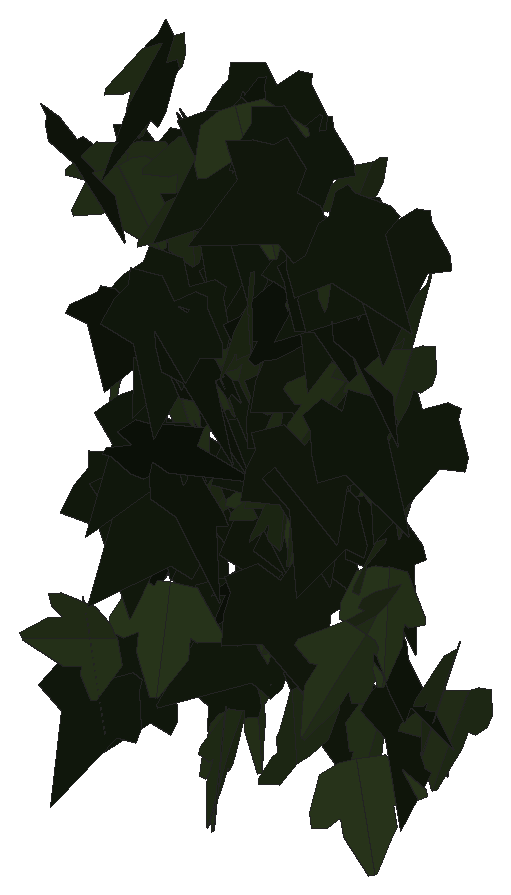
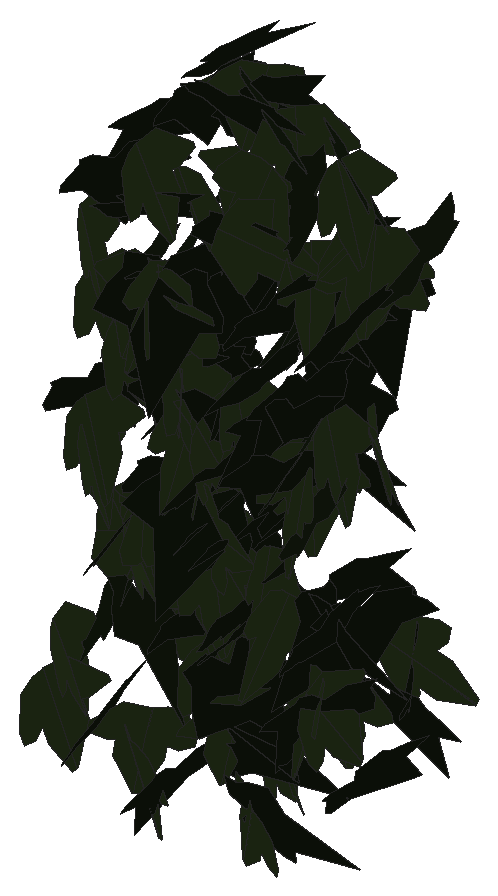
# SketchUp Ruby script. Lengths in inches.
U = 1.inch
M = Sketchup.active_model
def pt(a) = Geom::Point3d.new(a.map { |v| v * U })
def face(e, loops, mat)
  f = e.add_face(loops[0].map { |a| pt(a) })
  loops[1..].each { |l| e.add_face(l.map { |a| pt(a) }).erase! }
  f.material = f.back_material = mat if mat
  f
end
# faces: each face lists its corners as indices into pts; further lists are holes
def faces(e, pts, list, mat = nil) = list.each { |f| face(e, (f[0].is_a?(Array) ? f : [f]).map { |l| l.map { |i| pts[i] } }, mat) }
# xy, xz, yz: faces in a plane at the given z, y or x. An outline is a flat list of corners, or four numbers for a rectangle; further outlines are holes
def ring(l) = l.size == 4 ? [[l[0], l[1]], [l[2], l[1]], [l[2], l[3]], [l[0], l[3]]] : l.each_slice(2).to_a
def flat(e, list, mat, &to3) = list.each { |f| face(e, (f[0].is_a?(Array) ? f : [f]).map { |l| ring(l).map { |u, v| to3.(u, v) } }, mat) }
def xy(e, z, list, mat = nil) = flat(e, list, mat) { |x, y| [x, y, z] }
def xz(e, y, list, mat = nil) = flat(e, list, mat) { |x, z| [x, y, z] }
def yz(e, x, list, mat = nil) = flat(e, list, mat) { |y, z| [x, y, z] }
def lines(e, pts, list) = list.each { |a, b| e.add_line(pt(pts[a]), pt(pts[b])) }
# prism: a flat outline (further loops are holes) pulled along v
def prism(e, loops, v, mat = nil)
  f = face(e, loops, mat); d = Geom::Vector3d.new(v.map { |x| x * U })
  f.pushpull(f.normal.samedirection?(d) ? d.length : -d.length)
end
def box(e, o, s, mat = nil) = prism(e, [[o, [o[0] + s[0], o[1], o[2]], [o[0] + s[0], o[1] + s[1], o[2]], [o[0], o[1] + s[1], o[2]]]], [0, 0, s[2]], mat)
def at(x, y, z, deg = 0) = Geom::Transformation.translation(pt([x, y, z])) * Geom::Transformation.rotation(ORIGIN, Z_AXIS, deg.degrees)
def axes(o, x, y, z) = Geom::Transformation.new([*x, 0, *y, 0, *z, 0, *pt(o).to_a, 1])
def part(name) = M.definitions.add(name)
# library, detail: a bought-in or finely detailed component or shape, given as its bounding box
def library(name, o, s) = part(name).tap { |d| box(d.entities, o, s) }
def detail(e, o, s) = box(e.add_group.entities, o, s)
def put(e, d, t, mat = nil) = e.add_instance(d, t).tap { |i| i.material = mat if mat }
def group(e, t, mat = nil) = e.add_group.tap { |g| g.transformation = t; g.material = mat if mat }.entities
root = M.entities
M.materials.add("efeu1").color = [18, 25, 13]
M.materials.add("efeu2").color = [43, 57, 29]
c1 = part("ivyleaf_10")
p = [[0,0.5,-0.03],[-0.0625,2.02,-0.43],[-0.19,2.01,-0.46],[-0.54,1.05,-0.29],[-0.52,0.625,-0.18],[-0.83,0.76,-0.28],
  [-1.16,0.64,-0.33],[-1.15,0.33,-0.24],[-0.77,-0.39,0.02],[-0.3,-0.51,0.16],[0.04,-0.48,0.23],[-0.02,2.01,-0.4375],
  [-0.06,2.01,-0.43],[0.04,-0.49,0.23],[0.67,-0.49,0.14],[1.38,0.36,-0.2],[1.375,0.51,-0.24],[0.81,0.65,-0.19],
  [0.62,0.59,-0.15],[0.6,1.09,-0.28],[0.5,1.23,-0.31]]
faces(c1.entities,p,[[0,1,2,3,4,5,6,7,8,9,10],[11,12,0,13,14,15,16,17,18,19,20]],"efeu2")
c2 = part("ivyleaf_9")
p = [[1.54,2.16,1.25],[1.36,2.04,1.19],[-0.21,0.99,0.68],[-0.71,1.11,0.82],[-0.85,0.86,0.67],[-0.8,0.17,0.21],
  [-0.9,-0.01,0.1],[-0.67,-0.16,-0.02],[-0.08,-0.08,-0.05],[-0.03,-0.6,-0.4],[0.65,-0.88,-0.66],[0.83,-0.6,-0.49],
  [1.29,-0.42,-0.43],[1.8125,-0.07,-0.26],[1.21,0.44,0.15]]
faces(c2.entities,p,[[0,1,2,3,4,5,6,7,8,9,10,11,12,13,14]],"efeu1")
put(root,c1,axes([10.84,223.45,235.51],[0.02548,-0.41018,0.28478],[0.04221,-0.28236,-0.41048],[0.49756,0.04496,0.02023]))
put(root,c2,axes([10.51,222.08,240.66],[0.18822,-0.39499,0.24198],[0.16985,-0.18415,-0.43271],[0.43096,0.24509,0.06485]))
put(root,c1,axes([10.89,223.15,238.77],[0.04724,-0.49773,-0.006],[-0.00088,0.00594,-0.49996],[0.49776,0.04725,-0.00031]))
put(root,c1,axes([11.29,221.38,235.1875],[0.17508,0.01809,-0.46799],[-0.45924,0.10468,-0.16776],[0.09191,0.48858,0.05327]))
put(root,c2,axes([11.35,222.68,236.02],[-0.27745,0.22546,0.34956],[-0.26223,0.23136,-0.35736],[-0.32289,-0.38163,-0.01014]))
put(root,c1,axes([10.84,222.45,238.39],[0.34561,-0.29172,0.2132],[0.16573,-0.13418,-0.45225],[0.32107,0.38327,0.00395]))
put(root,c2,axes([10.78,223.09,240.23],[0.09676,-0.48882,-0.0412],[-0.00215,0.04157,-0.49826],[0.49054,0.0966,0.00594]))
put(root,c2,axes([10.89,222.64,236.41],[-0.18069,-0.44824,-0.12818],[0.05611,0.11556,-0.48322],[0.46282,-0.18901,0.00854]))
put(root,c2,axes([10.79,223.46,235.625],[0.0421,-0.43866,-0.23623],[0.04754,0.23953,-0.43631],[0.49595,0.01428,0.06188]))
put(root,c1,axes([11.03,223.36,235.61],[-0.38254,0.31627,0.06032],[-0.04509,0.04013,-0.49634],[-0.3188,-0.38518,-0.00218]))
put(root,c2,axes([11,222.59,234.2],[-0.18711,-0.40957,0.21735],[-0.052,-0.21436,-0.44871],[0.46074,-0.19053,0.03762]))
put(root,c2,axes([10.9,223.36,236.46],[0.01066,-0.49178,0.08967],[-0.01623,-0.08999,-0.49157],[0.49962,0.00757,-0.01788]))
put(root,c1,axes([11.12,222.19,240.65],[-0.39827,-0.30148,-0.02208],[0.01989,0.0103,-0.4995],[0.30163,-0.39875,0.00379]))
put(root,c1,axes([11.14,222.65,241.67],[-0.03559,-0.49633,0.04884],[0.00728,-0.04948,-0.49749],[0.49868,-0.0347,0.01075]))
put(root,c1,axes([11.11,222.17,240.39],[-0.35194,-0.31525,-0.16357],[0.14773,0.07947,-0.47102],[0.32297,-0.37987,0.03721]))
put(root,c2,axes([11.36,222.57,236.07],[-0.06999,0.10256,-0.48434],[-0.28778,0.3896,0.12408],[0.40285,0.29613,0.00449]))
put(root,c2,axes([11.01,223.32,237.77],[0.07513,-0.36679,0.33139],[0.13299,-0.30784,-0.37087],[0.4761,0.14387,0.0513]))
put(root,c2,axes([11.7,223.52,233.92],[-0.31021,0.15343,0.36087],[-0.32922,0.14808,-0.34596],[-0.21303,-0.45225,0.00915]))
put(root,c2,axes([11.37,221.51,234.61],[-0.45437,-0.12225,-0.16912],[0.1684,0.02449,-0.47015],[0.12324,-0.48421,0.01892]))
put(root,c1,axes([11.47,223.05,237.92],[-0.41018,0.24847,0.14148],[-0.12293,0.07011,-0.47955],[-0.25814,-0.42819,0.00357]))
put(root,c2,axes([11.48,222.32,241.83],[-0.42375,0.15045,-0.21864],[0.20508,-0.07586,-0.44965],[-0.16847,-0.47076,0.00259]))
put(root,c1,axes([11.53,222.84,238.07],[-0.421,-0.25867,0.07647],[-0.06549,-0.03947,-0.49412],[0.26166,-0.42607,-0.00065]))
put(root,c1,axes([11.34,222.52,235.1],[0.47007,0.17038,0.00269],[0.00214,0.00197,-0.49999],[-0.17039,0.47007,0.00112]))
put(root,c2,axes([11.5,222.37,236.4],[-0.26805,-0.37411,0.19543],[-0.06401,-0.1928,-0.45687],[0.4172,-0.26994,0.05546]))
put(root,c2,axes([11.34,223.1,239.26],[0.10277,-0.38413,-0.30312],[-0.06428,0.29645,-0.39747],[0.48508,0.12067,0.01155]))
put(root,c2,axes([11.2,221.4,235.17],[0.10419,-0.08708,-0.48121],[0.46944,-0.12002,0.12336],[-0.13699,-0.47751,0.05674]))
put(root,c1,axes([11.54,223.25,236.35],[-0.07687,-0.38054,-0.31508],[0.11176,0.29721,-0.38623],[0.48125,-0.12981,0.03936]))
put(root,c2,axes([11.45,223.21,238.9375],[0.09899,-0.3626,-0.32973],[0.0401,0.34125,-0.36323],[0.48846,0.04547,0.09665]))
put(root,c2,axes([11.53,223.23,238.24],[-0.1301,-0.41783,-0.24186],[0.10378,0.22043,-0.43662],[0.47149,-0.16381,0.02937]))
put(root,c2,axes([11.82,221.88,237.74],[-0.48579,-0.0778,-0.08917],[0.09055,-0.00181,-0.49173],[0.07619,-0.49391,0.01585]))
put(root,c2,axes([11.52,223.19,238.13],[0.03974,-0.3783,0.32452],[0.03619,-0.3225,-0.38038],[0.4971,0.05372,0.00175]))
put(root,c1,axes([11.68,222.3125,238.125],[-0.48655,0.04075,-0.10777],[0.10295,-0.05621,-0.48605],[-0.05173,-0.49516,0.04631]))
put(root,c2,axes([11.96,223.44,234.66],[-0.44214,-0.18738,0.13927],[-0.1315,-0.04659,-0.48014],[0.19292,-0.46121,-0.00808]))
put(root,c1,axes([11.77,223.1875,236.82],[0.04076,-0.43502,-0.24311],[0.03143,0.24568,-0.43434],[0.49734,0.02012,0.04737]))
put(root,c1,axes([11.81,222.37,240.28],[-0.10591,-0.47674,-0.10723],[0.01577,0.10633,-0.48831],[0.4884,-0.10681,-0.00748]))
put(root,c1,axes([11.67,223.57,233.89],[0.36571,-0.17378,0.29335],[0.27919,-0.09433,-0.40393],[0.19573,0.45924,0.02804]))
put(root,c2,axes([12.04,221.09,239.6],[0.22806,0.29386,-0.33412],[-0.20359,-0.26493,-0.37197],[-0.39565,0.30572,-0.00119]))
put(root,c2,axes([12.14,223.38,235.53],[-0.14157,0.39536,-0.27138],[-0.00204,-0.28346,-0.41188],[-0.47954,-0.11551,0.08187]))
put(root,c2,axes([11.9,223.06,240.01],[-0.06871,-0.48727,0.0886],[-0.00063,-0.08936,-0.49195],[0.49526,-0.06772,0.01167]))
put(root,c2,axes([12.25,223.34,235.95],[-0.11499,-0.48033,0.07788],[0.01734,0.07593,0.4939],[-0.48629,0.11629,-0.00081]))
put(root,c2,axes([11.84,222.38,241.13],[0.44335,-0.22332,-0.05972],[-0.05211,0.0293,-0.49641],[0.22522,0.4464,0.00271]))
put(root,c1,axes([12.42,222.86,240.65],[0.14389,0.08329,-0.47155],[-0.47746,-0.01255,-0.14791],[-0.03647,0.49285,0.07593]))
put(root,c1,axes([12.01,223.44,235.1],[0.16365,0.46864,0.05992],[0.00654,0.06116,-0.4962],[-0.47241,0.16319,0.01389]))
put(root,c2,axes([12.17,221.84,239.54],[-0.40783,-0.26544,-0.11495],[0.10084,0.05578,-0.48654],[0.27112,-0.42003,0.00804]))
put(root,c1,axes([12.5625,223.24,237.01],[0.08937,-0.00659,0.4919],[-0.48188,0.09947,0.08888],[-0.09903,-0.48996,0.01143]))
put(root,c2,axes([12.05,223.01,239.15],[0.15848,-0.43802,-0.18173],[-0.02721,0.18289,-0.46455],[0.47344,0.15714,0.03414]))
put(root,c1,axes([12.34,222.97,238.65],[0.03883,-0.49819,-0.01743],[0.00051,0.01752,-0.49969],[0.49849,0.03878,0.00187]))
put(root,c2,axes([12.2,223.34,235.86],[-0.0899,-0.44301,0.21367],[0.00605,-0.21819,-0.44984],[0.49182,-0.07829,0.04459]))
put(root,c1,axes([12.39,223.4,235.54],[-0.20066,-0.41968,0.18331],[-0.00122,-0.19964,-0.45841],[0.45797,-0.18442,0.07909]))
put(root,c2,axes([12.21,223.23,237.07],[0.02918,-0.49184,-0.08508],[0.01466,0.08603,-0.49232],[0.49893,0.02624,0.01944]))
put(root,c1,axes([12.47,223.26,236.625],[-0.15938,-0.47378,0.01133],[-0.0037,-0.01071,-0.49987],[0.4739,-0.15942,-0.0001]))
put(root,c1,axes([12.35,222.62,241.22],[-0.46665,0.10009,-0.14905],[0.13531,-0.07676,-0.47518],[-0.11801,-0.48383,0.04456]))
put(root,c1,axes([12.24,222.31,233.93],[0.29802,-0.249,0.31493],[0.25425,-0.18649,-0.38804],[0.31071,0.39143,0.01545]))
put(root,c2,axes([12.19,220.99,238.03],[0.42036,0.15167,0.22427],[0.20486,0.0926,-0.44661],[-0.17701,0.46735,0.01571]))
put(root,c1,axes([12.52,223.24,236.64],[-0.32542,-0.37456,0.06166],[0.02624,-0.10322,-0.48853],[0.3787,-0.31472,0.08683]))
put(root,c1,axes([12.54,221.75,241.45],[-0.28648,-0.40978,-0.00337],[0.00194,0.00276,-0.49999],[0.40979,-0.28648,0]))
put(root,c1,axes([12.41,222.31,234.01],[0.12891,-0.40923,0.25674],[0.1434,-0.22133,-0.42479],[0.46132,0.18315,0.06031]))
put(root,c2,axes([12.47,222.76,240.62],[-0.34704,-0.2344,-0.27316],[0.22642,0.1528,-0.41879],[0.27981,-0.41438,0.00009]))
put(root,c2,axes([12.3,221.65,237.35],[0.19597,-0.44556,0.11432],[0.05896,-0.0989,-0.48656],[0.4562,0.20418,0.01378]))
put(root,c2,axes([12.51,221.19,239.75],[-0.087,-0.49152,0.0289],[0.0062,-0.03043,-0.49903],[0.49233,-0.08648,0.01139]))
put(root,c2,axes([12.66,223.2,237.4],[0.30201,0.39839,-0.00861],[-0.05714,0.0326,-0.49565],[-0.39437,0.30037,0.06522]))
put(root,c1,axes([12.73,223.1,236.92],[-0.06092,-0.49148,0.06879],[-0.01639,-0.06728,-0.49518],[0.496,-0.06259,-0.00792]))
put(root,c1,axes([12.72,223.06,238.03],[0.07347,-0.44124,0.22341],[0.05732,-0.21675,-0.44692],[0.49124,0.09129,0.01874]))
put(root,c2,axes([12.53,223.19,237.82],[0.12921,-0.46086,-0.14462],[-0.00778,0.1477,-0.47762],[0.48295,0.12568,0.031]))
put(root,c2,axes([12.49,221.39,239.08],[0.35007,-0.35578,-0.02955],[-0.01918,0.02259,-0.49912],[0.35649,0.35059,0.00217]))
put(root,c2,axes([12.51,221.35,239.27],[0.27087,-0.41733,0.04961],[0.03053,-0.03933,-0.49751],[0.41916,0.27255,0.00418]))
put(root,c2,axes([12.67,222.18,241.89],[-0.30074,-0.12828,-0.37828],[0.39862,-0.12679,-0.27392],[-0.02564,-0.46634,0.17853]))
put(root,c1,axes([12.8,223.19,236.96],[-0.06748,0.43614,-0.235],[-0.05861,-0.24254,-0.43329],[-0.49195,-0.03093,0.08386]))
put(root,c2,axes([12.6,223.22,237.125],[0.1337,-0.47945,-0.0474],[-0.00301,0.04836,-0.49765],[0.48178,0.13336,0.01004]))
put(root,c1,axes([12.97,223.21,237.05],[-0.34111,-0.30692,0.1986],[-0.01705,-0.25797,-0.42797],[0.36517,-0.29874,0.16553]))
put(root,c2,axes([12.76,223.33,236.07],[-0.01074,-0.49353,0.07945],[-0.01487,-0.07912,-0.49348],[0.49966,-0.01296,-0.01297]))
put(root,c1,axes([12.7,222.28,241.05],[0.44842,0.09936,0.19761],[0.18547,0.07449,-0.45831],[-0.12051,0.48433,0.02995]))
put(root,c1,axes([12.91,222.85,237.37],[0.13847,-0.41704,-0.23854],[0.05263,0.25992,-0.42388],[0.47755,0.09228,0.11588]))
put(root,c1,axes([12.92,223.12,238.22],[-0.14774,-0.41674,-0.23345],[0.07754,0.22019,-0.44216],[0.47134,-0.16685,-0.00043]))
put(root,c2,axes([12.76,223.59,234.14],[0.12113,-0.46464,-0.13943],[-0.00241,0.14313,-0.47907],[0.4851,0.11673,0.03243]))
put(root,c1,axes([13.06,223.05,238.65],[0.01968,-0.4995,0.01053],[-0.0159,-0.01116,-0.49962],[0.49936,0.01933,-0.01632]))
put(root,c2,axes([13.18,221.77,241.58],[-0.33951,-0.30878,0.19845],[-0.15217,-0.1276,-0.45887],[0.33403,-0.37198,-0.00733]))
put(root,c2,axes([12.94,222.4,242.01],[-0.31891,-0.30864,-0.2303],[0.27558,0.02594,-0.41639],[0.26898,-0.39251,0.15357]))
put(root,c1,axes([13.17,223.2,236.92],[-0.36476,-0.33258,0.07965],[-0.01284,-0.10304,-0.4891],[0.34174,-0.35885,0.06663]))
put(root,c1,axes([13.16,223.1,238.55],[-0.36624,0.33536,0.05836],[-0.0993,-0.02326,-0.48949],[-0.32559,-0.37013,0.08364]))
put(root,c2,axes([13.03,223.17,238.55],[-0.31863,-0.21634,-0.31886],[0.27323,0.16489,-0.38491],[0.2717,-0.41953,0.01314]))
put(root,c1,axes([13.04,221.68,241.89],[0.31381,0.37076,0.11857],[0.07411,0.0926,-0.48573],[-0.38214,0.32243,0.00316]))
put(root,c2,axes([12.99,222.125,239.14],[0.13825,-0.01823,0.48016],[0.40863,0.26733,-0.1075],[-0.25281,0.42214,0.08881]))
put(root,c2,axes([13.36,222.95,239.73],[0.17749,0.46253,-0.06756],[-0.01839,-0.0653,-0.49538],[-0.46708,0.17833,-0.00616]))
put(root,c2,axes([13.25,222.97,237.58],[-0.2102,-0.44286,-0.09843],[0.02762,0.09579,-0.48996],[0.45283,-0.21142,-0.01581]))
put(root,c1,axes([13.37,222,237.53],[0.11563,-0.47086,-0.12216],[-0.00083,0.12538,-0.48403],[0.48645,0.11214,0.02821]))
put(root,c1,axes([13.42,222.9375,239.7],[-0.12971,-0.38107,-0.29659],[0.10432,0.27773,-0.40247],[0.47148,-0.16629,0.00745]))
put(root,c1,axes([13.47,222.98,239.39],[0.0993,-0.48695,-0.05499],[0.0079,0.05769,-0.4966],[0.48998,0.09775,0.01916]))
put(root,c2,axes([13.28,222.71,238.74],[-0.12887,-0.39143,-0.28315],[0.11642,0.25925,-0.41138],[0.46887,-0.17196,0.02432]))
put(root,c1,axes([13.3,222.95,239.35],[0.43107,0.19461,0.1622],[0.12086,0.12337,-0.46923],[-0.22265,0.44374,0.05932]))
put(root,c2,axes([13.3,222.07,236.23],[-0.0444,-0.41939,-0.26859],[0.08431,0.25943,-0.41903],[0.49084,-0.0825,0.04768]))
put(root,c2,axes([13.45,222.9375,239.87],[-0.21282,-0.45204,-0.01918],[0.00103,0.02071,-0.49957],[0.45244,-0.21268,-0.00789]))
put(root,c1,axes([13.5,223.31,233.91],[0.40811,-0.28882,-0.0054],[-0.00436,0.00319,-0.49997],[0.28884,0.40813,0.00008]))
put(root,c1,axes([13.57,222.61,238.46],[-0.02261,-0.35836,0.34795],[0.00621,-0.34848,-0.3585],[0.49945,-0.01189,0.0202]))
put(root,c1,axes([13.71,222.14,240.5],[0.40056,-0.23955,-0.17935],[-0.14375,0.1088,-0.46637],[0.26246,0.42518,0.0183]))
put(root,c2,axes([13.53,222.07,241.82],[-0.06506,-0.48821,-0.08615],[-0.00492,0.08752,-0.49226],[0.49572,-0.06321,-0.01619]))
put(root,c1,axes([13.56,222.99,239.73],[0.45971,0.09467,0.17236],[0.13009,0.18225,-0.44706],[-0.14748,0.45587,0.14293]))
put(root,c1,axes([13.8,222.81,241.05],[0.00936,-0.48429,0.12401],[0.00459,-0.12394,-0.48437],[0.49989,0.0102,0.00212]))
put(root,c2,axes([13.5625,222.2,240],[0.30026,-0.3922,-0.07757],[-0.0504,0.0591,-0.49393],[0.39661,0.30444,-0.00404]))
put(root,c2,axes([14.04,222.57,235.37],[-0.22782,0.445,0.00861],[-0.0039,0.00768,-0.49993],[-0.44506,-0.22785,-0.00002]))
put(root,c1,axes([13.91,223.03,238.89],[0.00915,-0.4725,0.16328],[0.00382,-0.16324,-0.47259],[0.4999,0.0099,0.00063]))
put(root,c1,axes([13.83,221.71,234.56],[-0.05331,-0.46357,-0.17962],[-0.02261,-0.1782,0.46662],[-0.49664,0.05787,-0.00196]))
put(root,c1,axes([13.96,220.6,240.45],[0.12513,-0.39278,-0.28296],[-0.05682,0.27833,-0.41147],[0.48074,0.13513,0.02502]))
put(root,c1,axes([13.88,222.92,236.37],[0.22865,-0.40165,0.19078],[0.10525,-0.15954,-0.46203],[0.43202,0.25145,0.01159]))
put(root,c2,axes([14.05,221.3,241.625],[-0.30436,-0.23178,0.32193],[-0.12164,-0.3317,-0.35381],[0.37758,-0.29369,0.14553]))
put(root,c2,axes([13.78,221.86,238.14],[-0.03464,-0.46575,-0.17855],[0.04342,0.17549,-0.46617],[0.4969,-0.0478,0.02829]))
put(root,c2,axes([13.81,223.125,236.71],[0.19224,-0.46156,0.00164],[-0.00737,-0.00485,-0.49992],[0.46151,0.19219,-0.00867]))
put(root,c2,axes([14.22,222.6,240.33],[-0.41934,-0.23095,0.14427],[-0.05765,-0.18361,-0.46148],[0.26613,-0.40367,0.12736]))
put(root,c1,axes([13.98,222.53,233.85],[0.35862,0.33603,0.09208],[0.06293,0.0675,-0.49141],[-0.34269,0.36405,0.00612]))
put(root,c2,axes([13.98,222,237.61],[-0.07871,-0.43486,0.23388],[0.03857,-0.24153,-0.43609],[0.49226,-0.0506,0.07157]))
put(root,c2,axes([13.99,223.44,234.28],[0.04533,-0.45302,0.20669],[0.0074,-0.20691,-0.45512],[0.49789,0.04432,-0.01206]))
put(root,c1,axes([14.22,223.24,237.59],[0.14515,-0.47818,0.01658],[0.00907,-0.01457,-0.49971],[0.47838,0.14536,0.00444]))
put(root,c1,axes([14.27,223.17,237.85],[-0.04735,-0.49684,0.03013],[0.00219,-0.03047,-0.49907],[0.49775,-0.04713,0.00507]))
put(root,c1,axes([14.4375,222.56,236.125],[-0.08,0.20009,-0.45118],[-0.30857,-0.377,-0.11248],[-0.3852,0.26045,0.18381]))
put(root,c2,axes([14.03,222.49,239.49],[0.23169,-0.42246,0.13359],[0.05251,-0.12351,-0.48165],[0.43996,0.23722,-0.01286]))
put(root,c1,axes([14.33,221.97,235.8],[-0.13394,-0.32466,0.35589],[0.04572,-0.37629,-0.32606],[0.47955,-0.0548,0.13049]))
put(root,c2,axes([14.26,222.67,235.51],[0.37994,-0.20746,-0.25022],[-0.20085,0.15278,-0.43165],[0.25556,0.42851,0.03275]))
put(root,c2,axes([14.375,223.07,238.26],[-0.25656,-0.4291,-0.00662],[0.00762,0.00315,-0.49993],[0.42909,-0.25663,0.00493]))
put(root,c1,axes([14.53,223.5625,234.51],[-0.11959,-0.46824,0.12827],[-0.00303,-0.13138,-0.48242],[0.48548,-0.11616,0.02859]))
put(root,c2,axes([14.22,221.77,241.13],[0.108,-0.37075,-0.31762],[0.08321,0.33452,-0.36218],[0.48105,0.02537,0.13396]))
put(root,c2,axes([14.42,222.5625,240.78],[-0.16138,-0.45866,-0.11656],[0.028,0.11368,-0.4861],[0.47241,-0.16342,-0.01101]))
put(root,c1,axes([14.51,223.37,235.08],[0.16466,-0.45935,0.10901],[0.03984,-0.10152,-0.48796],[0.47043,0.16938,0.00317]))
put(root,c1,axes([14.38,222.46,236.37],[0.48101,-0.04752,0.12795],[0.12568,-0.0286,-0.4831],[0.05323,0.49691,-0.01557]))
put(root,c1,axes([14.59,222.54,239.16],[-0.11234,-0.47257,0.11858],[0.00991,-0.12388,-0.48431],[0.48712,-0.10647,0.0372]))
put(root,c1,axes([14.65,222.75,239.93],[0.17099,-0.46892,-0.02958],[-0.00698,0.02894,-0.49911],[0.4698,0.1711,0.00335]))
put(root,c2,axes([14.48,221.68,238.89],[0.209,-0.40005,-0.21512],[-0.05069,0.21478,-0.44867],[0.45139,0.20935,0.04922]))
